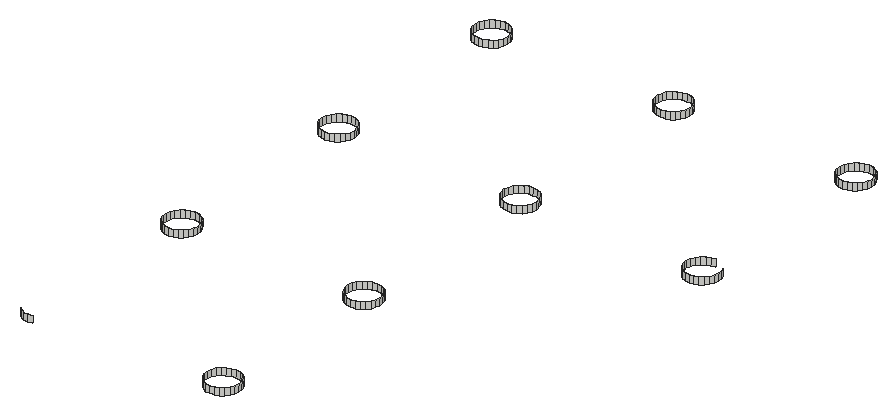
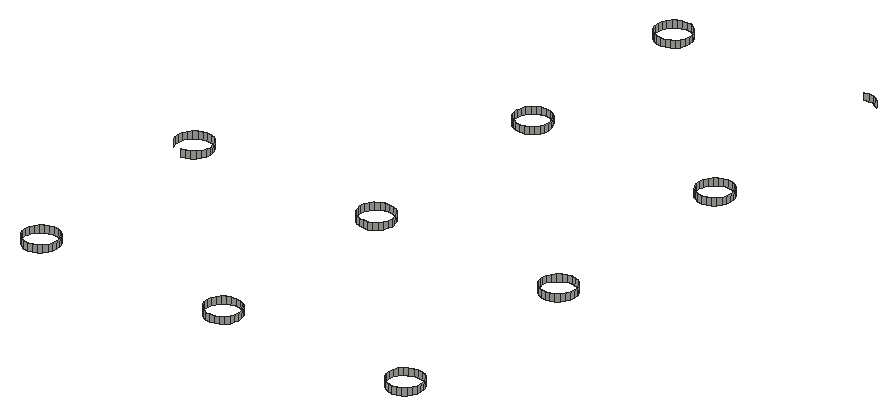
# SketchUp Ruby script. Lengths in inches.
U = 1.inch
M = Sketchup.active_model
def pt(a) = Geom::Point3d.new(a.map { |v| v * U })
def face(e, loops, mat)
  f = e.add_face(loops[0].map { |a| pt(a) })
  loops[1..].each { |l| e.add_face(l.map { |a| pt(a) }).erase! }
  f.material = f.back_material = mat if mat
  f
end
# faces: each face lists its corners as indices into pts; further lists are holes
def faces(e, pts, list, mat = nil) = list.each { |f| face(e, (f[0].is_a?(Array) ? f : [f]).map { |l| l.map { |i| pts[i] } }, mat) }
# xy, xz, yz: faces in a plane at the given z, y or x. An outline is a flat list of corners, or four numbers for a rectangle; further outlines are holes
def ring(l) = l.size == 4 ? [[l[0], l[1]], [l[2], l[1]], [l[2], l[3]], [l[0], l[3]]] : l.each_slice(2).to_a
def flat(e, list, mat, &to3) = list.each { |f| face(e, (f[0].is_a?(Array) ? f : [f]).map { |l| ring(l).map { |u, v| to3.(u, v) } }, mat) }
def xy(e, z, list, mat = nil) = flat(e, list, mat) { |x, y| [x, y, z] }
def xz(e, y, list, mat = nil) = flat(e, list, mat) { |x, z| [x, y, z] }
def yz(e, x, list, mat = nil) = flat(e, list, mat) { |y, z| [x, y, z] }
def lines(e, pts, list) = list.each { |a, b| e.add_line(pt(pts[a]), pt(pts[b])) }
# prism: a flat outline (further loops are holes) pulled along v
def prism(e, loops, v, mat = nil)
  f = face(e, loops, mat); d = Geom::Vector3d.new(v.map { |x| x * U })
  f.pushpull(f.normal.samedirection?(d) ? d.length : -d.length)
end
def box(e, o, s, mat = nil) = prism(e, [[o, [o[0] + s[0], o[1], o[2]], [o[0] + s[0], o[1] + s[1], o[2]], [o[0], o[1] + s[1], o[2]]]], [0, 0, s[2]], mat)
def at(x, y, z, deg = 0) = Geom::Transformation.translation(pt([x, y, z])) * Geom::Transformation.rotation(ORIGIN, Z_AXIS, deg.degrees)
def axes(o, x, y, z) = Geom::Transformation.new([*x, 0, *y, 0, *z, 0, *pt(o).to_a, 1])
def part(name) = M.definitions.add(name)
# library, detail: a bought-in or finely detailed component or shape, given as its bounding box
def library(name, o, s) = part(name).tap { |d| box(d.entities, o, s) }
def detail(e, o, s) = box(e.add_group.entities, o, s)
def put(e, d, t, mat = nil) = e.add_instance(d, t).tap { |i| i.material = mat if mat }
def group(e, t, mat = nil) = e.add_group.tap { |g| g.transformation = t; g.material = mat if mat }.entities
root = M.entities
p = [[383.77,385.12,126],[382.48,385.29,126],[382.48,385.29,128.125],[383.77,385.12,128.125],[385.07,385.29,126],[385.07,385.29,128.125],
  [440.09,385.12,126],[438.79,385.29,126],[438.79,385.29,128.125],[440.09,385.12,128.125],[441.38,385.29,126],[441.38,385.29,128.125],
  [381.27,385.79,126],[381.27,385.79,128.125],[437.59,385.79,126],[437.59,385.79,128.125],[442.59,385.79,126],[442.59,385.79,128.125],
  [380.24,386.58,126],[380.24,386.58,128.125],[436.55,386.58,126],[436.55,386.58,128.125],[443.62,386.58,126],[443.62,386.58,128.125],
  [435.76,387.62,126],[435.76,387.62,128.125],[444.42,387.62,126],[444.42,387.62,128.125],[435.26,388.83,126],[435.26,388.83,128.125],
  [444.92,388.83,126],[444.92,388.83,128.125],[435.09,390.12,126],[435.09,390.12,128.125],[445.09,390.12,126],[445.09,390.12,128.125],
  [435.26,391.41,126],[435.26,391.41,128.125],[444.92,391.41,126],[444.92,391.41,128.125],[435.76,392.62,126],[435.76,392.62,128.125],
  [444.42,392.62,126],[444.42,392.62,128.125],[436.55,393.66,126],[436.55,393.66,128.125],[443.62,393.66,126],[443.62,393.66,128.125],
  [437.59,394.45,126],[437.59,394.45,128.125],[442.59,394.45,126],[442.59,394.45,128.125],[438.79,394.95,126],[438.79,394.95,128.125],
  [441.38,394.95,126],[441.38,394.95,128.125],[440.09,395.12,126],[440.09,395.12,128.125],[383.77,439.5625,126],[382.48,439.73,126],
  [382.48,439.73,128.125],[383.77,439.5625,128.125],[385.07,439.73,126],[385.07,439.73,128.125],[440.09,439.5625,126],[438.79,439.73,126],
  [438.79,439.73,128.125],[440.09,439.5625,128.125],[441.38,439.73,126],[441.38,439.73,128.125],[381.27,440.23,126],[381.27,440.23,128.125],
  [386.27,440.23,126],[386.27,440.23,128.125],[437.59,440.23,126],[437.59,440.23,128.125],[442.59,440.23,126],[442.59,440.23,128.125],
  [380.24,441.03,126],[380.24,441.03,128.125],[387.31,441.03,126],[387.31,441.03,128.125],[436.55,441.03,126],[436.55,441.03,128.125],
  [443.62,441.03,126],[443.62,441.03,128.125],[379.44,442.0625,126],[379.44,442.0625,128.125],[388.1,442.0625,126],[388.1,442.0625,128.125],
  [435.76,442.0625,126],[435.76,442.0625,128.125],[444.42,442.0625,126],[444.42,442.0625,128.125],[378.94,443.27,126],[378.94,443.27,128.125],
  [388.6,443.27,126],[388.6,443.27,128.125],[435.26,443.27,126],[435.26,443.27,128.125],[444.92,443.27,126],[444.92,443.27,128.125],
  [378.77,444.5625,126],[378.77,444.5625,128.125],[388.77,444.5625,126],[388.77,444.5625,128.125],[435.09,444.5625,126],[435.09,444.5625,128.125],
  [445.09,444.5625,126],[445.09,444.5625,128.125],[378.94,445.86,126],[378.94,445.86,128.125],[388.6,445.86,126],[388.6,445.86,128.125],
  [435.26,445.86,126],[435.26,445.86,128.125],[444.92,445.86,126],[444.92,445.86,128.125],[379.44,447.0625,126],[379.44,447.0625,128.125],
  [388.1,447.0625,126],[388.1,447.0625,128.125],[435.76,447.0625,126],[435.76,447.0625,128.125],[444.42,447.0625,126],[444.42,447.0625,128.125],
  [380.24,448.1,126],[380.24,448.1,128.125],[387.31,448.1,126],[387.31,448.1,128.125],[436.55,448.1,126],[436.55,448.1,128.125],
  [443.62,448.1,126],[443.62,448.1,128.125],[381.27,448.89,126],[381.27,448.89,128.125],[386.27,448.89,126],[386.27,448.89,128.125],
  [437.59,448.89,126],[437.59,448.89,128.125],[442.59,448.89,126],[442.59,448.89,128.125],[382.48,449.39,126],[382.48,449.39,128.125],
  [385.07,449.39,126],[385.07,449.39,128.125],[438.79,449.39,126],[438.79,449.39,128.125],[441.38,449.39,126],[441.38,449.39,128.125],
  [383.77,449.5625,126],[383.77,449.5625,128.125],[440.09,449.5625,126],[440.09,449.5625,128.125],[383.77,500.05,126],[382.48,500.22,126],
  [382.48,500.22,128.125],[383.77,500.05,128.125],[385.07,500.22,126],[385.07,500.22,128.125],[440.09,500.05,126],[438.79,500.22,126],
  [438.79,500.22,128.125],[440.09,500.05,128.125],[441.38,500.22,126],[441.38,500.22,128.125],[496.4,500.05,126],[495.11,500.22,126],
  [495.11,500.22,128.125],[496.4,500.05,128.125],[497.69,500.22,126],[497.69,500.22,128.125],[381.27,500.72,126],[381.27,500.72,128.125],
  [386.27,500.72,126],[386.27,500.72,128.125],[437.59,500.72,126],[437.59,500.72,128.125],[442.59,500.72,126],[442.59,500.72,128.125],
  [493.9,500.72,126],[493.9,500.72,128.125],[498.9,500.72,126],[498.9,500.72,128.125],[380.24,501.52,126],[380.24,501.52,128.125],
  [387.31,501.52,126],[387.31,501.52,128.125],[436.55,501.52,126],[436.55,501.52,128.125],[443.62,501.52,126],[443.62,501.52,128.125],
  [492.86,501.52,126],[492.86,501.52,128.125],[499.93,501.52,126],[499.93,501.52,128.125],[379.44,502.55,126],[379.44,502.55,128.125],
  [388.1,502.55,126],[388.1,502.55,128.125],[435.76,502.55,126],[435.76,502.55,128.125],[444.42,502.55,126],[444.42,502.55,128.125],
  [492.07,502.55,126],[492.07,502.55,128.125],[500.73,502.55,126],[500.73,502.55,128.125],[378.94,503.76,126],[378.94,503.76,128.125],
  [388.6,503.76,126],[388.6,503.76,128.125],[435.26,503.76,126],[435.26,503.76,128.125],[444.92,503.76,126],[444.92,503.76,128.125],
  [491.57,503.76,126],[491.57,503.76,128.125],[501.23,503.76,126],[501.23,503.76,128.125],[378.77,505.05,126],[378.77,505.05,128.125],
  [388.77,505.05,126],[388.77,505.05,128.125],[435.09,505.05,126],[435.09,505.05,128.125],[445.09,505.05,126],[445.09,505.05,128.125],
  [491.4,505.05,126],[491.4,505.05,128.125],[501.4,505.05,126],[501.4,505.05,128.125],[378.94,506.35,126],[378.94,506.35,128.125],
  [388.6,506.35,126],[388.6,506.35,128.125],[435.26,506.35,126],[435.26,506.35,128.125],[444.92,506.35,126],[444.92,506.35,128.125],
  [491.57,506.35,126],[491.57,506.35,128.125],[501.23,506.35,126],[501.23,506.35,128.125],[379.44,507.55,126],[379.44,507.55,128.125],
  [388.1,507.55,126],[388.1,507.55,128.125],[435.76,507.55,126],[435.76,507.55,128.125],[444.42,507.55,126],[444.42,507.55,128.125],
  [492.07,507.55,126],[492.07,507.55,128.125],[500.73,507.55,126],[500.73,507.55,128.125],[380.24,508.59,126],[380.24,508.59,128.125],
  [387.31,508.59,126],[387.31,508.59,128.125],[436.55,508.59,126],[436.55,508.59,128.125],[443.62,508.59,126],[443.62,508.59,128.125],
  [492.86,508.59,126],[492.86,508.59,128.125],[381.27,509.38,126],[381.27,509.38,128.125],[386.27,509.38,126],[386.27,509.38,128.125],
  [437.59,509.38,126],[437.59,509.38,128.125],[442.59,509.38,126],[442.59,509.38,128.125],[493.9,509.38,126],[493.9,509.38,128.125],
  [382.48,509.88,126],[382.48,509.88,128.125],[385.07,509.88,126],[385.07,509.88,128.125],[438.79,509.88,126],[438.79,509.88,128.125],
  [441.38,509.88,126],[441.38,509.88,128.125],[495.11,509.88,126],[495.11,509.88,128.125],[383.77,510.05,126],[383.77,510.05,128.125],
  [440.09,510.05,126],[440.09,510.05,128.125],[496.4,510.05,126],[496.4,510.05,128.125],[383.77,559.33,126],[382.48,559.5,126],
  [382.48,559.5,128.125],[383.77,559.33,128.125],[385.07,559.5,126],[385.07,559.5,128.125],[440.09,559.33,126],[438.79,559.5,126],
  [438.79,559.5,128.125],[440.09,559.33,128.125],[441.38,559.5,126],[441.38,559.5,128.125],[496.4,559.33,126],[495.11,559.5,126],
  [495.11,559.5,128.125],[496.4,559.33,128.125],[497.69,559.5,126],[497.69,559.5,128.125],[381.27,560,126],[381.27,560,128.125],
  [386.27,560,126],[386.27,560,128.125],[437.59,560,126],[437.59,560,128.125],[442.59,560,126],[442.59,560,128.125],
  [493.9,560,126],[493.9,560,128.125],[498.9,560,126],[498.9,560,128.125],[380.24,560.79,126],[380.24,560.79,128.125],
  [387.31,560.79,126],[387.31,560.79,128.125],[436.55,560.79,126],[436.55,560.79,128.125],[443.62,560.79,126],[443.62,560.79,128.125],
  [492.86,560.79,126],[492.86,560.79,128.125],[499.93,560.79,126],[499.93,560.79,128.125],[379.44,561.83,126],[379.44,561.83,128.125],
  [388.1,561.83,126],[388.1,561.83,128.125],[435.76,561.83,126],[435.76,561.83,128.125],[444.42,561.83,126],[444.42,561.83,128.125],
  [492.07,561.83,126],[492.07,561.83,128.125],[500.73,561.83,126],[500.73,561.83,128.125],[378.94,563.03,126],[378.94,563.03,128.125],
  [388.6,563.03,126],[388.6,563.03,128.125],[435.26,563.03,126],[435.26,563.03,128.125],[444.92,563.03,126],[444.92,563.03,128.125],
  [491.57,563.03,126],[491.57,563.03,128.125],[501.23,563.03,126],[501.23,563.03,128.125],[378.77,564.33,126],[378.77,564.33,128.125],
  [388.77,564.33,126],[388.77,564.33,128.125],[435.09,564.33,126],[435.09,564.33,128.125],[445.09,564.33,126],[445.09,564.33,128.125],
  [491.4,564.33,126],[491.4,564.33,128.125],[501.4,564.33,126],[501.4,564.33,128.125],[378.94,565.62,126],[378.94,565.62,128.125],
  [388.6,565.62,126],[388.6,565.62,128.125],[435.26,565.62,126],[435.26,565.62,128.125],[444.92,565.62,126],[444.92,565.62,128.125],
  [491.57,565.62,126],[491.57,565.62,128.125],[501.23,565.62,126],[501.23,565.62,128.125],[379.44,566.83,126],[379.44,566.83,128.125],
  [388.1,566.83,126],[388.1,566.83,128.125],[435.76,566.83,126],[435.76,566.83,128.125],[444.42,566.83,126],[444.42,566.83,128.125],
  [492.07,566.83,126],[492.07,566.83,128.125],[500.73,566.83,126],[500.73,566.83,128.125],[380.24,567.86,126],[380.24,567.86,128.125],
  [387.31,567.86,126],[387.31,567.86,128.125],[436.55,567.86,126],[436.55,567.86,128.125],[443.62,567.86,126],[443.62,567.86,128.125],
  [492.86,567.86,126],[492.86,567.86,128.125],[499.93,567.86,126],[499.93,567.86,128.125],[381.27,568.66,126],[381.27,568.66,128.125],
  [386.27,568.66,126],[386.27,568.66,128.125],[437.59,568.66,126],[437.59,568.66,128.125],[442.59,568.66,126],[442.59,568.66,128.125],
  [493.9,568.66,126],[493.9,568.66,128.125],[498.9,568.66,126],[498.9,568.66,128.125],[382.48,569.16,126],[382.48,569.16,128.125],
  [385.07,569.16,126],[385.07,569.16,128.125],[438.79,569.16,126],[438.79,569.16,128.125],[441.38,569.16,126],[441.38,569.16,128.125],
  [495.11,569.16,126],[495.11,569.16,128.125],[497.69,569.16,126],[497.69,569.16,128.125],[383.77,569.33,126],[383.77,569.33,128.125],
  [440.09,569.33,126],[440.09,569.33,128.125],[496.4,569.33,126],[496.4,569.33,128.125]]
faces(root,p,[[0,1,2,3],[4,0,3,5],[6,7,8,9],[10,6,9,11],[1,12,13,2],[7,14,15,8],[16,10,11,17],[12,18,19,13],
  [14,20,21,15],[22,16,17,23],[20,24,25,21],[26,22,23,27],[24,28,29,25],[30,26,27,31],[28,32,33,29],[34,30,31,35],
  [32,36,37,33],[38,34,35,39],[36,40,41,37],[42,38,39,43],[40,44,45,41],[46,42,43,47],[44,48,49,45],[50,46,47,51],
  [48,52,53,49],[54,50,51,55],[52,56,57,53],[56,54,55,57],[58,59,60,61],[62,58,61,63],[64,65,66,67],[68,64,67,69],
  [59,70,71,60],[72,62,63,73],[65,74,75,66],[76,68,69,77],[70,78,79,71],[80,72,73,81],[74,82,83,75],[84,76,77,85],
  [78,86,87,79],[88,80,81,89],[82,90,91,83],[92,84,85,93],[86,94,95,87],[96,88,89,97],[90,98,99,91],[100,92,93,101],
  [94,102,103,95],[104,96,97,105],[98,106,107,99],[108,100,101,109],[102,110,111,103],[112,104,105,113],[106,114,115,107],[116,108,109,117],
  [110,118,119,111],[120,112,113,121],[114,122,123,115],[124,116,117,125],[118,126,127,119],[128,120,121,129],[122,130,131,123],[132,124,125,133],
  [126,134,135,127],[136,128,129,137],[130,138,139,131],[140,132,133,141],[134,142,143,135],[144,136,137,145],[138,146,147,139],[148,140,141,149],
  [142,150,151,143],[150,144,145,151],[146,152,153,147],[152,148,149,153],[154,155,156,157],[158,154,157,159],[160,161,162,163],[164,160,163,165],
  [166,167,168,169],[170,166,169,171],[155,172,173,156],[174,158,159,175],[161,176,177,162],[178,164,165,179],[167,180,181,168],[182,170,171,183],
  [172,184,185,173],[186,174,175,187],[176,188,189,177],[190,178,179,191],[180,192,193,181],[194,182,183,195],[184,196,197,185],[198,186,187,199],
  [188,200,201,189],[202,190,191,203],[192,204,205,193],[206,194,195,207],[196,208,209,197],[210,198,199,211],[200,212,213,201],[214,202,203,215],
  [204,216,217,205],[218,206,207,219],[208,220,221,209],[222,210,211,223],[212,224,225,213],[226,214,215,227],[216,228,229,217],[230,218,219,231],
  [220,232,233,221],[234,222,223,235],[224,236,237,225],[238,226,227,239],[228,240,241,229],[242,230,231,243],[232,244,245,233],[246,234,235,247],
  [236,248,249,237],[250,238,239,251],[240,252,253,241],[254,242,243,255],[244,256,257,245],[258,246,247,259],[248,260,261,249],[262,250,251,263],
  [252,264,265,253],[256,266,267,257],[268,258,259,269],[260,270,271,261],[272,262,263,273],[264,274,275,265],[266,276,277,267],[278,268,269,279],
  [270,280,281,271],[282,272,273,283],[274,284,285,275],[276,286,287,277],[286,278,279,287],[280,288,289,281],[288,282,283,289],[284,290,291,285],
  [292,293,294,295],[296,292,295,297],[298,299,300,301],[302,298,301,303],[304,305,306,307],[308,304,307,309],[293,310,311,294],[312,296,297,313],
  [299,314,315,300],[316,302,303,317],[305,318,319,306],[320,308,309,321],[310,322,323,311],[324,312,313,325],[314,326,327,315],[328,316,317,329],
  [318,330,331,319],[332,320,321,333],[322,334,335,323],[336,324,325,337],[326,338,339,327],[340,328,329,341],[330,342,343,331],[344,332,333,345],
  [334,346,347,335],[348,336,337,349],[338,350,351,339],[352,340,341,353],[342,354,355,343],[356,344,345,357],[346,358,359,347],[360,348,349,361],
  [350,362,363,351],[364,352,353,365],[354,366,367,355],[368,356,357,369],[358,370,371,359],[372,360,361,373],[362,374,375,363],[376,364,365,377],
  [366,378,379,367],[380,368,369,381],[370,382,383,371],[384,372,373,385],[374,386,387,375],[388,376,377,389],[378,390,391,379],[392,380,381,393],
  [382,394,395,383],[396,384,385,397],[386,398,399,387],[400,388,389,401],[390,402,403,391],[404,392,393,405],[394,406,407,395],[408,396,397,409],
  [398,410,411,399],[412,400,401,413],[402,414,415,403],[416,404,405,417],[406,418,419,407],[420,408,409,421],[410,422,423,411],[424,412,413,425],
  [414,426,427,415],[428,416,417,429],[418,430,431,419],[430,420,421,431],[422,432,433,423],[432,424,425,433],[426,434,435,427],[434,428,429,435]])
